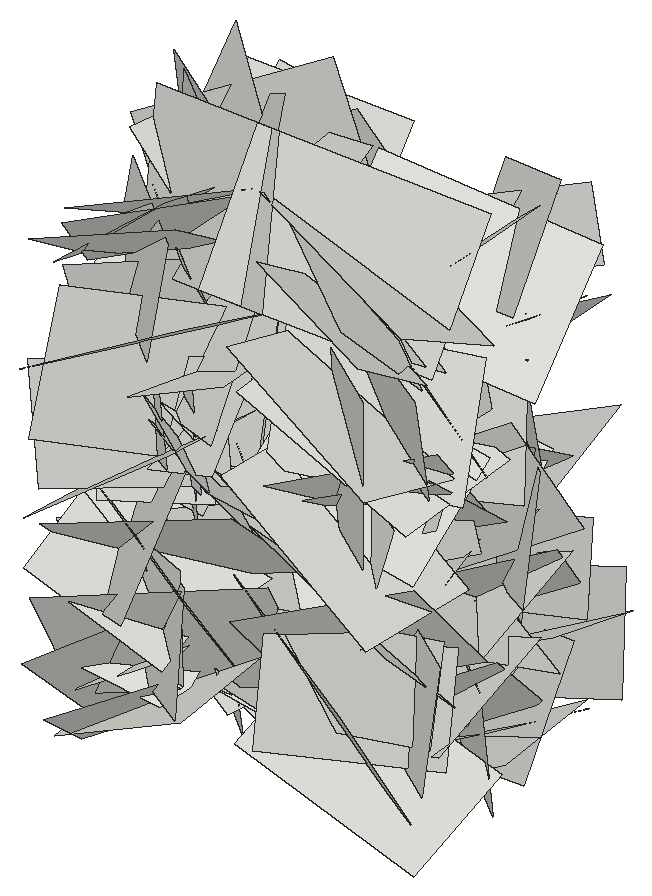
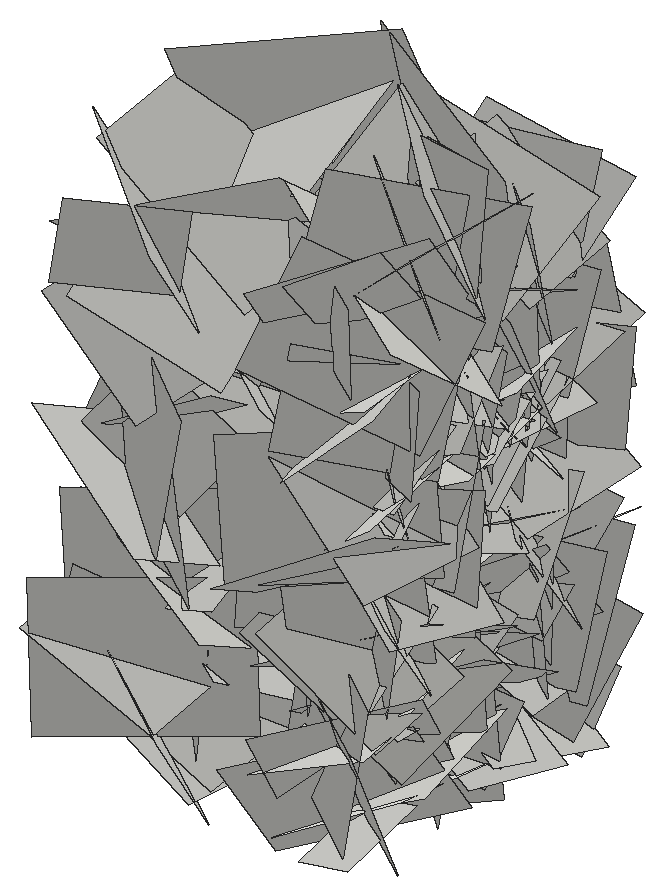
# SketchUp Ruby script. Lengths in inches.
U = 1.inch
M = Sketchup.active_model
def pt(a) = Geom::Point3d.new(a.map { |v| v * U })
def face(e, loops, mat)
  f = e.add_face(loops[0].map { |a| pt(a) })
  loops[1..].each { |l| e.add_face(l.map { |a| pt(a) }).erase! }
  f.material = f.back_material = mat if mat
  f
end
# faces: each face lists its corners as indices into pts; further lists are holes
def faces(e, pts, list, mat = nil) = list.each { |f| face(e, (f[0].is_a?(Array) ? f : [f]).map { |l| l.map { |i| pts[i] } }, mat) }
# xy, xz, yz: faces in a plane at the given z, y or x. An outline is a flat list of corners, or four numbers for a rectangle; further outlines are holes
def ring(l) = l.size == 4 ? [[l[0], l[1]], [l[2], l[1]], [l[2], l[3]], [l[0], l[3]]] : l.each_slice(2).to_a
def flat(e, list, mat, &to3) = list.each { |f| face(e, (f[0].is_a?(Array) ? f : [f]).map { |l| ring(l).map { |u, v| to3.(u, v) } }, mat) }
def xy(e, z, list, mat = nil) = flat(e, list, mat) { |x, y| [x, y, z] }
def xz(e, y, list, mat = nil) = flat(e, list, mat) { |x, z| [x, y, z] }
def yz(e, x, list, mat = nil) = flat(e, list, mat) { |y, z| [x, y, z] }
def lines(e, pts, list) = list.each { |a, b| e.add_line(pt(pts[a]), pt(pts[b])) }
# prism: a flat outline (further loops are holes) pulled along v
def prism(e, loops, v, mat = nil)
  f = face(e, loops, mat); d = Geom::Vector3d.new(v.map { |x| x * U })
  f.pushpull(f.normal.samedirection?(d) ? d.length : -d.length)
end
def box(e, o, s, mat = nil) = prism(e, [[o, [o[0] + s[0], o[1], o[2]], [o[0] + s[0], o[1] + s[1], o[2]], [o[0], o[1] + s[1], o[2]]]], [0, 0, s[2]], mat)
def at(x, y, z, deg = 0) = Geom::Transformation.translation(pt([x, y, z])) * Geom::Transformation.rotation(ORIGIN, Z_AXIS, deg.degrees)
def axes(o, x, y, z) = Geom::Transformation.new([*x, 0, *y, 0, *z, 0, *pt(o).to_a, 1])
def part(name) = M.definitions.add(name)
# library, detail: a bought-in or finely detailed component or shape, given as its bounding box
def library(name, o, s) = part(name).tap { |d| box(d.entities, o, s) }
def detail(e, o, s) = box(e.add_group.entities, o, s)
def put(e, d, t, mat = nil) = e.add_instance(d, t).tap { |i| i.material = mat if mat }
def group(e, t, mat = nil) = e.add_group.tap { |g| g.transformation = t; g.material = mat if mat }.entities
root = M.entities
c1 = part("Component\#6")
p = [[0.01,0,0],[0,3.24,4.54],[4.32,3.24,4.54],[4.33,0,0]]
faces(c1.entities,p,[[0,1,2,3]])
put(root,c1,axes([410.71,147.32,10.4375],[-0.06119,-0.47987,-0.75245],[-0.01649,-0.75336,0.48165],[0.94584,-0.04418,-0.04028]))
put(root,c1,axes([414.68,136.7,5.12],[-0.11008,0.58852,-0.4619],[0.03608,-0.46213,-0.59646],[-0.7922,-0.10282,0.03702]))
put(root,c1,axes([414.68,135.6875,17.375],[0.11773,0.10526,0.9962],[0.108,0.99592,-0.11659],[-1.05635,0.11356,0.09911]))
put(root,c1,axes([414.68,144.39,10.35],[0.12238,0.87118,-0.30871],[0.00416,-0.31157,-0.87778],[-0.97971,0.1075,-0.04229]))
put(root,c1,axes([410.71,139.94,18.75],[-0.02341,-0.9115,0.17831],[-0.09444,0.17962,0.90714],[0.97996,-0.00447,0.09169]))
put(root,c1,axes([414.68,141.47,13.3125],[0.15098,-0.93805,0.13539],[0.00567,0.13771,0.94846],[-1.00463,-0.1402,0.0257]))
put(root,c1,axes([414.68,143.17,8.1],[-0.04482,0.75985,0.07181],[-0.00358,0.07173,-0.76102],[-0.80902,-0.04241,-0.00061]))
put(root,c1,axes([414.68,139.62,7.21],[0.15609,-0.9187,-0.23757],[0.00588,-0.23958,0.92989],[-1.00583,-0.14396,-0.03143]))
put(root,c1,axes([410.71,145.65,3.28],[0.1646,0.60158,-0.34623],[0.0091,-0.35642,-0.61544],[0.73568,-0.13018,0.08507]))
put(root,c1,axes([414.68,141.35,5.69],[-0.05421,0.52298,-0.48745],[-0.04158,-0.49001,-0.52162],[-0.75668,-0.01054,0.06359]))
put(root,c1,axes([410.71,143.03,2.65],[-0.18528,-0.93043,-0.12384],[0.14778,-0.15031,0.9325],[0.98392,-0.15263,-0.16338]))
put(root,c1,axes([414.68,149.3125,5.88],[0.15882,-0.57412,-0.80425],[0.08368,-0.80389,0.58857],[-1.04409,-0.15176,-0.07517]))
put(root,c1,axes([414.68,141.5625,11.54],[0.13399,-0.80117,0.38482],[-0.02481,0.38556,0.81039],[-0.9418,-0.12414,0.0334]))
put(root,c1,axes([414.68,147.06,19.23],[0.16196,0.05609,-0.92604],[-0.00217,-0.93849,-0.05718],[-0.9834,0.01131,-0.15239]))
put(root,c1,axes([410.71,141.85,18.04],[-0.12661,-0.3078,1.12748],[-0.24587,1.11705,0.28038],[1.21422,0.1941,0.17434]))
put(root,c1,axes([414.68,142.57,12.97],[0.12959,-0.66136,0.5647],[-0.03976,0.56572,0.67067],[-0.92097,-0.11748,0.0505]))
put(root,c1,axes([414.68,147.56,10.64],[-0.00206,-0.13591,-0.77504],[0.03252,-0.77447,0.13573],[-0.83344,-0.02988,0.00721]))
put(root,c1,axes([410.71,143.95,11.7],[-0.02215,-0.88691,-0.38082],[-0.08723,-0.37788,0.88459],[1.0194,-0.05161,0.06742]))
put(root,c1,axes([410.71,144.05,16.5],[0.02895,-0.76847,-0.41691],[-0.01722,-0.41749,0.76847],[0.92657,0.01625,0.02731]))
put(root,c1,axes([414.68,143.33,2.25],[-0.06381,-0.71847,0.0034],[0.02834,0.00117,0.7205],[-0.76106,0.06028,0.02655]))
put(root,c1,axes([410.71,147.01,9.44],[-0.18802,-1.10018,-0.17062],[-0.06994,-0.16208,1.11371],[1.17806,-0.18521,0.03889]))
put(root,c1,axes([410.71,143.66,16.18],[0.1105,0.58717,-0.52568],[0.01323,-0.53143,-0.59111],[0.83529,-0.06926,0.0789]))
put(root,c1,axes([410.71,145.52,18.22],[-0.02537,0.1253,-0.85934],[0.08829,-0.85537,-0.12704],[0.91628,0.08589,-0.01155]))
put(root,c1,axes([414.68,146.8125,4.55],[0.17148,-0.83232,0.10491],[-0.08015,0.09194,0.84603],[-0.88562,-0.16948,-0.05625]))
put(root,c1,axes([410.71,139.77,3.95],[0.11908,-0.78329,-0.0515],[0.03618,-0.0471,0.79084],[0.83129,0.11425,-0.02704]))
put(root,c1,axes([410.71,143.76,15.19],[0.09057,0.86782,-0.29614],[-0.1091,-0.28647,-0.86917],[0.96584,-0.11373,-0.07041]))
put(root,c1,axes([414.68,138.58,20.36],[0.30182,0.3301,1.08442],[0.18064,1.09293,-0.37743],[-1.1879,0.25007,0.21813]))
put(root,c1,axes([410.71,142.07,24.73],[-0.13514,0.30002,-0.93652],[0.09595,-0.93677,-0.31242],[1.03799,0.12565,-0.09305]))
put(root,c1,axes([414.68,143.53,7.33],[0.11895,-0.88372,0.009],[0.0734,0.01784,0.88799],[-0.93392,-0.11115,0.07094]))
put(root,c1,axes([410.71,139.41,15.5],[0.07329,-0.02436,0.98546],[-0.16551,0.97513,0.03506],[1.03171,0.15816,-0.06438]))
put(root,c1,axes([414.68,142.73,15.75],[0.26089,1.021,-0.12695],[0.10549,-0.15355,-1.04195],[-1.08548,0.23047,-0.13178]))
put(root,c1,axes([414.68,136.74,12.93],[-0.11437,0.04247,0.59628],[-0.02624,0.60507,-0.04758],[-0.63311,-0.03275,-0.10574]))
put(root,c1,axes([410.71,145.52,15.88],[-0.20612,-0.51117,0.96001],[0.04532,0.97089,0.52562],[1.15198,-0.12966,0.1511]))
put(root,c1,axes([414.68,139.35,17.19],[-0.06054,-0.33637,0.61942],[0.0607,0.61718,0.34043],[-0.74468,0.07766,-0.02261]))
put(root,c1,axes([414.68,143.63,3.63],[-0.04495,-0.13338,0.65571],[-0.00407,0.65706,0.13341],[-0.70927,0.00468,-0.04233]))
put(root,c1,axes([414.68,140.67,1.375],[-0.09858,-0.02009,0.69473],[0.09996,0.69407,0.03269],[-0.72991,0.09776,-0.08935]))
put(root,c1,axes([410.71,137.55,18.4],[-0.05522,0.7917,0.38208],[0.20111,0.38385,-0.76951],[0.90986,-0.0368,0.19328]))
put(root,c1,axes([414.68,141.96,13.08],[-0.07799,-0.57044,-0.33182],[0.05167,-0.33766,0.56968],[-0.69762,0.03877,0.07929]))
put(root,c1,axes([410.71,146.4375,4.35],[-0.18242,-1.06895,0.55133],[-0.10581,0.56772,1.06956],[1.27052,-0.1062,0.16823]))
put(root,c1,axes([410.71,139.48,6.78],[0.1397,0.74364,0.31774],[0.04551,0.31504,-0.75514],[0.85599,-0.13812,-0.01171]))
put(root,c1,axes([414.68,147.44,21.48],[-0.11936,-0.32986,-0.48912],[0.02265,-0.49991,0.33221],[-0.62494,0.04489,0.10546]))
put(root,c1,axes([414.68,139.2,5.38],[0.02645,-0.5119,-0.36479],[-0.13209,-0.36186,0.49927],[-0.65307,0.05245,-0.11575]))
put(root,c1,axes([410.71,137.79,2.1],[-0.03475,-0.78477,0.75119],[-0.11687,0.75006,0.77877],[1.14558,0.05272,0.10224]))
put(root,c1,axes([414.68,141.75,2.2],[-0.07408,-0.19814,0.56205],[-0.01701,0.56632,0.19765],[-0.63148,0.00798,-0.07126]))
put(root,c1,axes([410.71,135.11,11.54],[-0.10699,0.00448,1.06975],[0.01257,1.07444,-0.00338],[1.13388,-0.01149,0.10098]))
put(root,c1,axes([414.68,139.97,19.34],[0.20036,-0.21311,0.82685],[0.01235,0.84743,0.21575],[-0.90502,-0.03562,0.186]))
put(root,c1,axes([410.71,145.41,21.68],[0.17174,-0.50133,-0.77339],[-0.12403,-0.79008,0.48764],[0.96905,-0.01227,0.19948]))
put(root,c1,axes([414.68,141.82,12.65],[-0.04235,0.31596,0.66399],[0.14644,0.65635,-0.30401],[-0.76557,0.10807,-0.09488]))
put(root,c1,axes([410.71,136.25,6.15],[0.02753,0.62765,0.83331],[-0.11118,0.83092,-0.62258],[1.10023,0.06826,-0.08377]))
put(root,c1,axes([410.71,142.09,4.39],[0.13266,-0.06807,0.83796],[0.05074,0.84639,0.06161],[0.88972,-0.03812,-0.12846]))
put(root,c1,axes([410.71,149.05,6.52],[-0.16475,-0.3536,-1.09271],[-0.00842,-1.10231,0.35784],[1.21738,-0.05548,-0.1454]))
put(root,c1,axes([414.68,138.56,10.4375],[0.05239,0.37979,0.51244],[-0.10197,0.51253,-0.37059],[-0.66837,-0.04842,0.0967]))
put(root,c1,axes([410.71,141.11,17.69],[0.01651,0.23078,-0.87547],[0.12637,-0.8685,-0.22682],[0.95135,0.11136,0.04532]))
put(root,c1,axes([410.71,140.66,10.67],[-0.05387,-0.70807,-1.02445],[-0.25854,-0.99979,0.70312],[1.29449,-0.22915,0.09779]))
put(root,c1,axes([414.68,145.32,5.58],[-0.01721,-0.24816,-0.73855],[0.187,-0.7207,0.23828],[-0.80443,-0.16223,0.07119]))
put(root,c1,axes([410.71,139.9,15.42],[0.08068,-0.00169,-0.87701],[0.08263,-0.87681,0.00845],[0.92595,0.07839,0.07566]))
put(root,c1,axes([414.68,139.99,14.29],[-0.01199,-0.16574,0.68191],[0.09091,0.67656,0.16586],[-0.73829,0.086,0.00935]))
put(root,c1,axes([414.68,147.58,14.43],[0.15626,-0.88067,0.15465],[0.14549,0.17716,0.87807],[-0.93656,-0.11942,0.1622]))
put(root,c1,axes([414.68,138.3,10.21],[0.07821,-0.14386,0.79141],[0.12147,0.78851,0.13265],[-0.84394,0.10016,0.09244]))
put(root,c1,axes([410.71,142.2,15.72],[-0.2001,0.61396,-1.10583],[-0.10306,-1.12181,-0.60624],[1.33676,0.00542,-0.21228]))
put(root,c1,axes([410.71,141.25,1.55],[0.11713,-0.0063,1.0149],[-0.13715,1.01248,0.02037],[1.06704,0.13083,-0.10878]))
put(root,c1,axes([410.71,144.34,6.82],[-0.01542,0.93301,-0.17325],[0.14993,-0.1692,-0.92309],[0.99466,0.03997,0.13646]))
put(root,c1,axes([410.71,137.99,14.66],[-0.08461,-0.27233,0.9902],[0.1352,0.98287,0.28059],[1.08015,-0.14435,0.04245]))
put(root,c1,axes([410.71,142.29,19.52],[0.02505,0.60517,0.90894],[-0.1077,0.90642,-0.60085],[1.15246,0.07156,-0.07591]))
put(root,c1,axes([410.71,144.58,9.97],[0.16827,0.58944,-0.69808],[-0.0398,-0.70373,-0.60275],[0.96765,-0.13145,0.0966]))
put(root,c1,axes([414.68,139.8125,20.98],[-0.02151,0.52563,-0.34386],[0.05265,-0.34162,-0.52514],[-0.66372,-0.04413,-0.03051]))
put(root,c1,axes([414.68,142.6,14.22],[0.18899,-0.6396,-0.42028],[-0.00285,-0.43205,0.65638],[-0.81124,-0.14749,-0.10022]))
put(root,c1,axes([414.68,145.36,10.15],[0.14636,-0.64891,0.3527],[0.01811,0.36152,0.65845],[-0.78267,-0.11298,0.08119]))
put(root,c1,axes([414.68,145.42,18.19],[0.07853,-0.05807,0.70782],[0.06912,0.70921,0.05136],[-0.74963,0.05931,0.07889]))
put(root,c1,axes([410.71,146.45,10.34],[0.10559,0.05407,-0.92917],[0.0532,-0.93343,-0.04894],[0.98516,0.04461,0.10223]))
put(root,c1,axes([414.68,141.95,12.73],[0.09992,0.55515,0.3498],[-0.02862,0.35638,-0.5583],[-0.69495,0.06514,0.07329]))
put(root,c1,axes([410.71,137.63,3.85],[-0.23328,-0.07655,1.22947],[0.08564,1.24535,0.092],[1.30295,-0.09556,0.21407]))
put(root,c1,axes([410.71,137.89,18.97],[0.02244,-0.79516,0.48934],[0.22215,0.48102,0.77258],[0.96443,-0.0923,-0.18934]))
put(root,c1,axes([414.68,139.18,13.74],[0.11062,-0.13563,-0.63299],[-0.03095,-0.6415,0.13263],[-0.6855,0.00708,-0.10814]))
put(root,c1,axes([410.71,141.92,3.18],[0.02887,1.0089,0.10446],[0.06921,0.10254,-1.00735],[1.07292,-0.03376,0.06217]))
put(root,c1,axes([410.71,138.34,13.4],[0.1901,0.66514,0.65147],[-0.02496,0.66648,-0.67398],[0.98658,-0.1113,-0.14258]))
put(root,c1,axes([410.71,138.76,9.15],[0.08107,-0.07376,-0.93469],[0.12107,-0.93007,0.08274],[0.98644,0.12021,0.06666]))
put(root,c1,axes([410.71,139.52,8.83],[0.01584,-0.12995,-1.07448],[0.00128,-1.07458,0.12998],[1.14724,0.003,0.01469]))
put(root,c1,axes([410.71,137.41,10.49],[0.17918,0.96529,0.20208],[-0.06958,0.21558,-0.97489],[1.04307,-0.15144,-0.09975]))
put(root,c1,axes([410.71,141.07,4.77],[-0.0925,1.07709,-0.24358],[0.13853,-0.23255,-1.07513],[1.16232,0.11343,0.10875]))
put(root,c1,axes([410.71,143.54,11.83],[-0.01207,0.98557,0.48784],[0.03058,0.48797,-0.98515],[1.16528,-0.0026,0.03091]))
put(root,c1,axes([414.68,142.82,6.12],[-0.04161,-0.60559,-0.03198],[0.13563,-0.03959,0.59276],[-0.62835,0.03156,0.13006]))
put(root,c1,axes([410.71,142.72,8.07],[-0.13823,0.05764,1.30603],[-0.0986,1.30878,-0.06705],[1.38223,0.09912,0.12583]))
put(root,c1,axes([410.71,138.64,15.1],[-0.05154,1.07135,-0.23626],[0.10153,-0.23144,-1.06922],[1.15847,0.06794,0.08319]))
put(root,c1,axes([410.71,138.49,4.97],[-0.13436,1.04009,0.6085],[0.04809,0.61554,-1.04268],[1.27641,0.08629,0.10334]))
put(root,c1,axes([414.68,137.29,3.46],[0.14224,0.61257,0.15159],[-0.04066,0.16261,-0.62315],[-0.66768,0.1206,0.07024]))
put(root,c1,axes([410.71,137.21,11.6875],[-0.11385,0.72886,-0.88593],[0.14818,-0.87485,-0.7367],[1.20699,0.17615,0.00688]))
put(root,c1,axes([410.71,143.17,19.13],[0.20193,0.9279,-0.28366],[0.04691,-0.29708,-0.94209],[1.02744,-0.16881,0.09877]))
put(root,c1,axes([410.71,142.88,1.98],[0.0351,0.64216,0.95117],[0.00533,0.95147,-0.64254],[1.21649,-0.02269,-0.02463]))
put(root,c1,axes([410.71,137.64,18.89],[0.26376,-0.64139,0.69016],[0.02251,0.71746,0.65911],[0.99845,0.15326,-0.19718]))
put(root,c1,axes([410.71,140.93,18.6875],[-0.10901,-0.41314,-1.06231],[0.28274,-1.04573,0.38087],[1.17466,0.21337,-0.19026]))
put(root,c1,axes([410.71,141.75,2.91],[-0.11729,-1.19784,-0.30033],[0.11289,-0.30967,1.19584],[1.30414,-0.08092,-0.13053]))
put(root,c1,axes([410.71,143.08,17.68],[-0.06532,-0.13436,-1.17102],[0.13166,-1.16683,0.12734],[1.24247,0.11658,-0.07506]))
put(root,c1,axes([410.71,140.04,10.48],[-0.03722,-1.27767,0.05021],[-0.04996,0.05148,1.27723],[1.35446,-0.03321,0.04849]))
put(root,c1,axes([410.71,140.59,7.56],[-0.03383,1.06332,0.50099],[0.10932,0.50178,-1.05842],[1.24115,-0.01522,0.10688]))
put(root,c1,axes([410.71,137.94,15.45],[-0.03401,0.89045,-0.73196],[0.17038,-0.72163,-0.88493],[1.2099,0.12665,0.10405]))
put(root,c1,axes([410.71,146.96,20.2],[-0.19126,-1.0536,-0.82739],[0.10265,-0.84293,1.05228],[1.41631,-0.08119,-0.188]))
put(root,c1,axes([410.71,139.77,22.87],[0.12093,1.26112,-0.05281],[-0.18505,-0.03675,-1.25475],[1.32509,-0.12022,-0.17041]))
put(root,c1,axes([410.71,139.44,14.86],[-0.04621,-1.16691,0.31838],[0.12643,0.31289,1.16311],[1.27589,-0.07327,-0.10372]))
put(root,c1,axes([410.71,141.48,7.17],[0.20337,0.82379,-0.77749],[-0.08888,-0.77608,-0.84298],[1.19742,-0.19752,0.06948]))
put(root,c1,axes([410.71,138.37,16.22],[0.07456,0.76169,-0.90937],[0.0504,-0.91204,-0.76025],[1.25638,-0.00862,0.08446]))
put(root,c1,axes([410.71,144.3,10.94],[0.16969,-0.07735,1.18237],[-0.06112,1.19119,0.08573],[1.2545,0.0685,-0.15576]))
put(root,c1,axes([410.71,144.73,5.33],[0.04426,-1.02294,0.56209],[0.16257,0.56238,1.01208],[1.2265,-0.03763,-0.15444]))
put(root,c1,axes([410.71,141.11,14.91],[0.10517,-0.78429,-0.79452],[0.18451,-0.77703,0.78876],[1.16892,0.19321,-0.05302]))
put(root,c1,axes([410.71,134.59,13.6],[0.14779,0.17555,1.29716],[-0.16453,1.29751,-0.15892],[1.37773,0.13612,-0.15813]))
put(root,c1,axes([410.71,148.13,7.79],[0.13698,0.11741,-1.23467],[-0.05668,-1.23967,-0.12348],[1.31343,-0.06574,0.12344]))
put(root,c1,axes([410.71,139.3125,6.46],[-0.05297,-0.89114,0.82127],[0.332,0.78454,0.87035],[1.24093,-0.24794,-0.1978]))
put(root,c1,axes([410.71,142.16,14.375],[-0.02255,-1.26636,-0.09652],[0.2141,-0.09868,1.25016],[1.3291,-0.00559,-0.20302]))
put(root,c1,axes([410.71,141.32,18.93],[-0.00931,-1.12138,0.55372],[0.26786,0.54072,1.09906],[1.29833,-0.1196,-0.22278]))
put(root,c1,axes([410.71,140.96,14.21],[0.1647,-0.56811,1.02456],[0.16232,1.03452,0.5504],[1.23116,-0.0604,-0.20963]))
put(root,c1,axes([410.71,137.06,3.09],[0.11239,-0.69918,1.17187],[0.18512,1.17269,0.68387],[1.43458,-0.09655,-0.18006]))
put(root,c1,axes([410.71,141.18,23.91],[0.20239,-0.45291,-1.29893],[0.24414,-1.28235,0.48098],[1.43758,0.28153,0.10118]))
put(root,c1,axes([424.49,141.18,23.91],[-0.20239,-0.45291,-1.29893],[-0.24414,-1.28235,0.48098],[-1.43758,0.28153,0.10118]))
put(root,c1,axes([424.49,137.06,3.09],[-0.11239,-0.69918,1.17187],[-0.18512,1.17269,0.68387],[-1.43458,-0.09655,-0.18006]))
put(root,c1,axes([424.49,140.96,14.21],[-0.1647,-0.56811,1.02456],[-0.16232,1.03452,0.5504],[-1.23116,-0.0604,-0.20963]))
put(root,c1,axes([424.49,141.32,18.93],[0.00931,-1.12138,0.55372],[-0.26786,0.54072,1.09906],[-1.29833,-0.1196,-0.22278]))
put(root,c1,axes([424.49,142.16,14.375],[0.02255,-1.26636,-0.09652],[-0.2141,-0.09868,1.25016],[-1.3291,-0.00559,-0.20302]))
put(root,c1,axes([424.49,139.3125,6.46],[0.05297,-0.89114,0.82127],[-0.332,0.78454,0.87035],[-1.24093,-0.24794,-0.1978]))
put(root,c1,axes([424.49,148.13,7.79],[-0.13698,0.11741,-1.23467],[0.05668,-1.23967,-0.12348],[-1.31343,-0.06574,0.12344]))
put(root,c1,axes([424.49,134.59,13.6],[-0.14779,0.17555,1.29716],[0.16453,1.29751,-0.15892],[-1.37773,0.13612,-0.15813]))
put(root,c1,axes([424.49,141.11,14.91],[-0.10517,-0.78429,-0.79452],[-0.18451,-0.77703,0.78876],[-1.16892,0.19321,-0.05302]))
put(root,c1,axes([424.49,144.73,5.33],[-0.04426,-1.02294,0.56209],[-0.16257,0.56238,1.01208],[-1.2265,-0.03763,-0.15444]))
put(root,c1,axes([424.49,144.3,10.94],[-0.16969,-0.07735,1.18237],[0.06112,1.19119,0.08573],[-1.2545,0.0685,-0.15576]))
put(root,c1,axes([424.49,138.37,16.22],[-0.07456,0.76169,-0.90937],[-0.0504,-0.91204,-0.76025],[-1.25638,-0.00862,0.08446]))
put(root,c1,axes([424.49,141.48,7.17],[-0.20337,0.82379,-0.77749],[0.08888,-0.77608,-0.84298],[-1.19742,-0.19752,0.06948]))
put(root,c1,axes([424.49,139.44,14.86],[0.04621,-1.16691,0.31838],[-0.12643,0.31289,1.16311],[-1.27589,-0.07327,-0.10372]))
put(root,c1,axes([424.49,139.77,22.87],[-0.12093,1.26112,-0.05281],[0.18505,-0.03675,-1.25475],[-1.32509,-0.12022,-0.17041]))
put(root,c1,axes([424.49,146.96,20.2],[0.19126,-1.0536,-0.82739],[-0.10265,-0.84293,1.05228],[-1.41631,-0.08119,-0.188]))
put(root,c1,axes([424.49,137.94,15.45],[0.03401,0.89045,-0.73196],[-0.17038,-0.72163,-0.88493],[-1.2099,0.12665,0.10405]))
put(root,c1,axes([424.49,140.59,7.56],[0.03383,1.06332,0.50099],[-0.10932,0.50178,-1.05842],[-1.24115,-0.01522,0.10688]))
put(root,c1,axes([424.49,140.04,10.48],[0.03722,-1.27767,0.05021],[0.04996,0.05148,1.27723],[-1.35446,-0.03321,0.04849]))
put(root,c1,axes([424.49,143.08,17.68],[0.06532,-0.13436,-1.17102],[-0.13166,-1.16683,0.12734],[-1.24247,0.11658,-0.07506]))
put(root,c1,axes([424.49,141.75,2.91],[0.11729,-1.19784,-0.30033],[-0.11289,-0.30967,1.19584],[-1.30414,-0.08092,-0.13053]))
put(root,c1,axes([424.49,140.93,18.6875],[0.10901,-0.41314,-1.06231],[-0.28274,-1.04573,0.38087],[-1.17466,0.21337,-0.19026]))
put(root,c1,axes([424.49,137.64,18.89],[-0.26376,-0.64139,0.69016],[-0.02251,0.71746,0.65911],[-0.99845,0.15326,-0.19718]))
put(root,c1,axes([424.49,142.88,1.98],[-0.0351,0.64216,0.95117],[-0.00533,0.95147,-0.64254],[-1.21649,-0.02269,-0.02463]))
put(root,c1,axes([424.49,143.17,19.13],[-0.20193,0.9279,-0.28366],[-0.04691,-0.29708,-0.94209],[-1.02744,-0.16881,0.09877]))
put(root,c1,axes([424.49,137.21,11.6875],[0.11385,0.72886,-0.88593],[-0.14818,-0.87485,-0.7367],[-1.20699,0.17615,0.00688]))
put(root,c1,axes([420.52,137.29,3.46],[-0.14224,0.61257,0.15159],[0.04066,0.16261,-0.62315],[0.66768,0.1206,0.07024]))
put(root,c1,axes([424.49,138.49,4.97],[0.13436,1.04009,0.6085],[-0.04809,0.61554,-1.04268],[-1.27641,0.08629,0.10334]))
put(root,c1,axes([424.49,138.64,15.1],[0.05154,1.07135,-0.23626],[-0.10153,-0.23144,-1.06922],[-1.15847,0.06794,0.08319]))
put(root,c1,axes([424.49,142.72,8.07],[0.13823,0.05764,1.30603],[0.0986,1.30878,-0.06705],[-1.38223,0.09912,0.12583]))
put(root,c1,axes([420.52,142.82,6.12],[0.04161,-0.60559,-0.03198],[-0.13563,-0.03959,0.59276],[0.62835,0.03156,0.13006]))
put(root,c1,axes([424.49,143.54,11.83],[0.01207,0.98557,0.48784],[-0.03058,0.48797,-0.98515],[-1.16528,-0.0026,0.03091]))
put(root,c1,axes([424.49,141.07,4.77],[0.0925,1.07709,-0.24358],[-0.13853,-0.23255,-1.07513],[-1.16232,0.11343,0.10875]))
put(root,c1,axes([424.49,137.41,10.49],[-0.17918,0.96529,0.20208],[0.06958,0.21558,-0.97489],[-1.04307,-0.15144,-0.09975]))
put(root,c1,axes([424.49,139.52,8.83],[-0.01584,-0.12995,-1.07448],[-0.00128,-1.07458,0.12998],[-1.14724,0.003,0.01469]))
put(root,c1,axes([424.49,138.76,9.15],[-0.08107,-0.07376,-0.93469],[-0.12107,-0.93007,0.08274],[-0.98644,0.12021,0.06666]))
put(root,c1,axes([424.49,138.34,13.4],[-0.1901,0.66514,0.65147],[0.02496,0.66648,-0.67398],[-0.98658,-0.1113,-0.14258]))
put(root,c1,axes([424.49,141.92,3.18],[-0.02887,1.0089,0.10446],[-0.06921,0.10254,-1.00735],[-1.07292,-0.03376,0.06217]))
put(root,c1,axes([420.52,139.18,13.74],[-0.11062,-0.13563,-0.63299],[0.03095,-0.6415,0.13263],[0.6855,0.00708,-0.10814]))
put(root,c1,axes([424.49,137.89,18.97],[-0.02244,-0.79516,0.48934],[-0.22215,0.48102,0.77258],[-0.96443,-0.0923,-0.18934]))
put(root,c1,axes([424.49,137.63,3.85],[0.23328,-0.07655,1.22947],[-0.08564,1.24535,0.092],[-1.30295,-0.09556,0.21407]))
put(root,c1,axes([420.52,141.95,12.73],[-0.09992,0.55515,0.3498],[0.02862,0.35638,-0.5583],[0.69495,0.06514,0.07329]))
put(root,c1,axes([424.49,146.45,10.34],[-0.10559,0.05407,-0.92917],[-0.0532,-0.93343,-0.04894],[-0.98516,0.04461,0.10223]))
put(root,c1,axes([420.52,145.42,18.19],[-0.07853,-0.05807,0.70782],[-0.06912,0.70921,0.05136],[0.74963,0.05931,0.07889]))
put(root,c1,axes([420.52,145.36,10.15],[-0.14636,-0.64891,0.3527],[-0.01811,0.36152,0.65845],[0.78267,-0.11298,0.08119]))
put(root,c1,axes([420.52,142.6,14.22],[-0.18899,-0.6396,-0.42028],[0.00285,-0.43205,0.65638],[0.81124,-0.14749,-0.10022]))
put(root,c1,axes([420.52,139.8125,20.98],[0.02151,0.52563,-0.34386],[-0.05265,-0.34162,-0.52514],[0.66372,-0.04413,-0.03051]))
put(root,c1,axes([424.49,144.58,9.97],[-0.16827,0.58944,-0.69808],[0.0398,-0.70373,-0.60275],[-0.96765,-0.13145,0.0966]))
put(root,c1,axes([424.49,142.29,19.52],[-0.02505,0.60517,0.90894],[0.1077,0.90642,-0.60085],[-1.15246,0.07156,-0.07591]))
put(root,c1,axes([424.49,137.99,14.66],[0.08461,-0.27233,0.9902],[-0.1352,0.98287,0.28059],[-1.08015,-0.14435,0.04245]))
put(root,c1,axes([424.49,144.34,6.82],[0.01542,0.93301,-0.17325],[-0.14993,-0.1692,-0.92309],[-0.99466,0.03997,0.13646]))
put(root,c1,axes([424.49,141.25,1.55],[-0.11713,-0.0063,1.0149],[0.13715,1.01248,0.02037],[-1.06704,0.13083,-0.10878]))
put(root,c1,axes([424.49,142.2,15.72],[0.2001,0.61396,-1.10583],[0.10306,-1.12181,-0.60624],[-1.33676,0.00542,-0.21228]))
put(root,c1,axes([420.52,138.3,10.21],[-0.07821,-0.14386,0.79141],[-0.12147,0.78851,0.13265],[0.84394,0.10016,0.09244]))
put(root,c1,axes([420.52,147.58,14.43],[-0.15626,-0.88067,0.15465],[-0.14549,0.17716,0.87807],[0.93656,-0.11942,0.1622]))
put(root,c1,axes([420.52,139.99,14.29],[0.01199,-0.16574,0.68191],[-0.09091,0.67656,0.16586],[0.73829,0.086,0.00935]))
